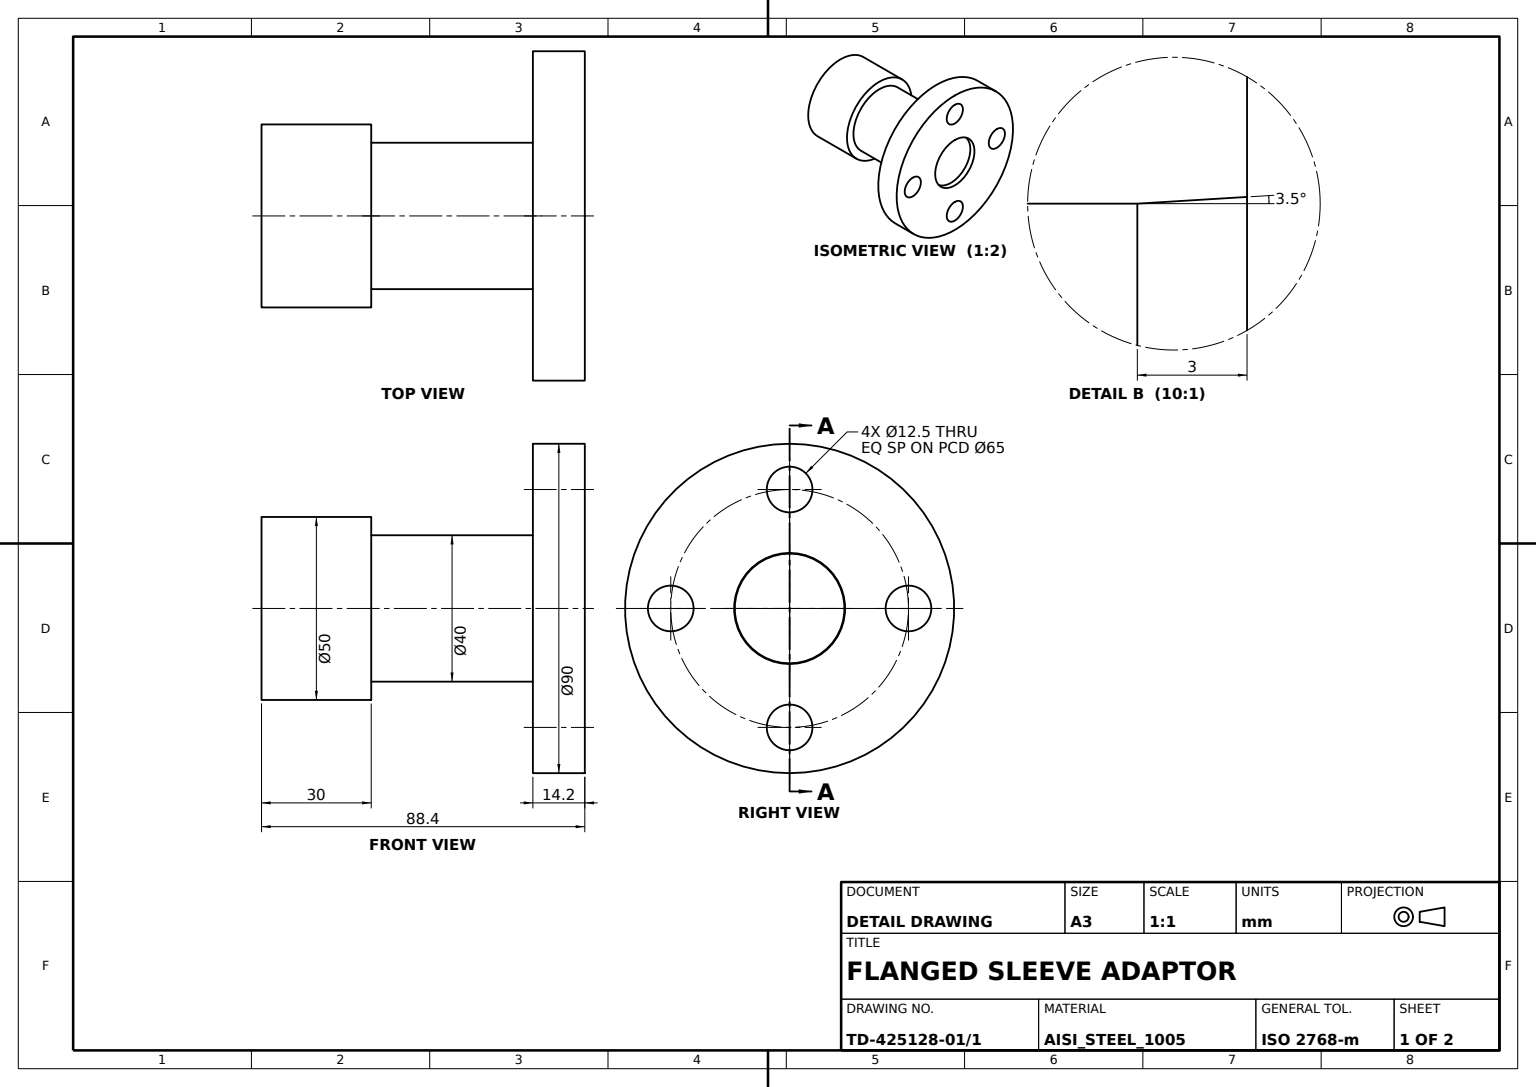
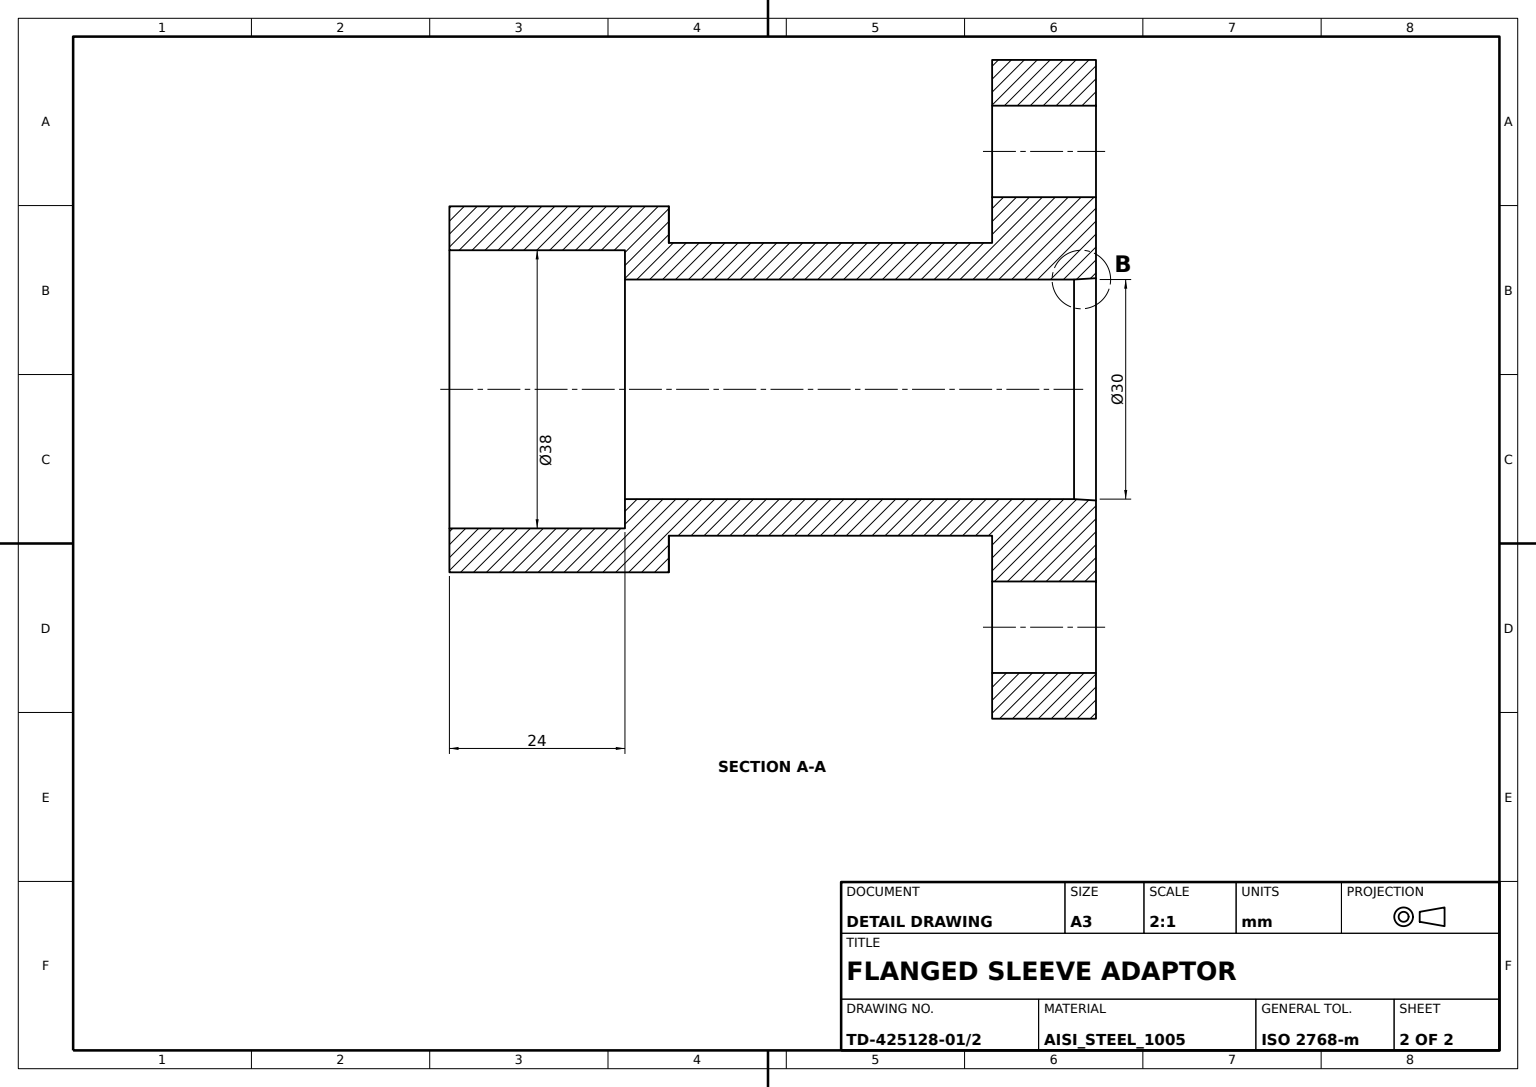
ISO-10303-21;
HEADER;
FILE_DESCRIPTION((''),'2;1');
FILE_NAME('','',(''),(''),'','','');
FILE_SCHEMA(('AUTOMOTIVE_DESIGN'));
ENDSEC;
DATA;
#1=APPLICATION_CONTEXT('');
#2=PRODUCT_CONTEXT('',#1,'mechanical');
#3=PRODUCT('','','',(#2));
#4=PRODUCT_DEFINITION_FORMATION('','',#3);
#5=PRODUCT_DEFINITION_CONTEXT('',#1,'design');
#6=PRODUCT_DEFINITION('','',#4,#5);
#7=PRODUCT_DEFINITION_SHAPE('','',#6);
#8=(LENGTH_UNIT()NAMED_UNIT(*)SI_UNIT(.MILLI.,.METRE.));
#9=(NAMED_UNIT(*)PLANE_ANGLE_UNIT()SI_UNIT($,.RADIAN.));
#10=(NAMED_UNIT(*)SI_UNIT($,.STERADIAN.)SOLID_ANGLE_UNIT());
#11=UNCERTAINTY_MEASURE_WITH_UNIT(LENGTH_MEASURE(0.005),#8,'distance_accuracy_value','');
#12=(GEOMETRIC_REPRESENTATION_CONTEXT(3)GLOBAL_UNCERTAINTY_ASSIGNED_CONTEXT((#11))GLOBAL_UNIT_ASSIGNED_CONTEXT((#8,#9,#10))REPRESENTATION_CONTEXT('',''));
#13=CARTESIAN_POINT('',(-58.4,0.,25.));
#14=VERTEX_POINT('',#13);
#15=CARTESIAN_POINT('',(-58.4,0.,0.));
#16=DIRECTION('',(-1.,0.,0.));
#17=DIRECTION('',(0.,0.,1.));
#18=AXIS2_PLACEMENT_3D('',#15,#16,#17);
#19=CIRCLE('',#18,25.);
#20=EDGE_CURVE('',#14,#14,#19,.T.);
#21=ORIENTED_EDGE('',*,*,#20,.F.);
#22=EDGE_LOOP('',(#21));
#23=FACE_BOUND('',#22,.T.);
#24=CARTESIAN_POINT('',(-58.4,0.,20.));
#25=VERTEX_POINT('',#24);
#26=CIRCLE('',#18,20.);
#27=EDGE_CURVE('',#25,#25,#26,.T.);
#28=ORIENTED_EDGE('',*,*,#27,.T.);
#29=EDGE_LOOP('',(#28));
#30=FACE_BOUND('',#29,.T.);
#31=AXIS2_PLACEMENT_3D('',#24,#16,#17);
#32=PLANE('',#31);
#33=ADVANCED_FACE('',(#23,#30),#32,.F.);
#34=CARTESIAN_POINT('',(-88.4,0.,25.));
#35=VERTEX_POINT('',#34);
#36=CARTESIAN_POINT('',(-88.4,0.,0.));
#37=AXIS2_PLACEMENT_3D('',#36,#16,#17);
#38=CIRCLE('',#37,25.);
#39=EDGE_CURVE('',#35,#35,#38,.T.);
#40=ORIENTED_EDGE('',*,*,#39,.F.);
#41=EDGE_LOOP('',(#40));
#42=FACE_BOUND('',#41,.T.);
#43=ORIENTED_EDGE('',*,*,#20,.T.);
#44=EDGE_LOOP('',(#43));
#45=FACE_BOUND('',#44,.T.);
#46=CARTESIAN_POINT('',(0.,0.,0.));
#47=AXIS2_PLACEMENT_3D('',#46,#16,#17);
#48=CYLINDRICAL_SURFACE('',#47,25.);
#49=ADVANCED_FACE('',(#42,#45),#48,.T.);
#50=CARTESIAN_POINT('',(0.,0.,45.));
#51=VERTEX_POINT('',#50);
#52=CIRCLE('',#47,45.);
#53=EDGE_CURVE('',#51,#51,#52,.T.);
#54=ORIENTED_EDGE('',*,*,#53,.T.);
#55=EDGE_LOOP('',(#54));
#56=FACE_BOUND('',#55,.T.);
#57=CARTESIAN_POINT('',(-14.2,0.,45.));
#58=VERTEX_POINT('',#57);
#59=CARTESIAN_POINT('',(-14.2,0.,0.));
#60=AXIS2_PLACEMENT_3D('',#59,#16,#17);
#61=CIRCLE('',#60,45.);
#62=EDGE_CURVE('',#58,#58,#61,.T.);
#63=ORIENTED_EDGE('',*,*,#62,.F.);
#64=EDGE_LOOP('',(#63));
#65=FACE_BOUND('',#64,.T.);
#66=CYLINDRICAL_SURFACE('',#47,45.);
#67=ADVANCED_FACE('',(#56,#65),#66,.T.);
#68=ORIENTED_EDGE('',*,*,#39,.T.);
#69=EDGE_LOOP('',(#68));
#70=FACE_BOUND('',#69,.T.);
#71=CARTESIAN_POINT('',(-88.4,19.,0.));
#72=VERTEX_POINT('',#71);
#73=DIRECTION('',(0.,1.,0.));
#74=AXIS2_PLACEMENT_3D('',#36,#16,#73);
#75=CIRCLE('',#74,19.);
#76=EDGE_CURVE('',#72,#72,#75,.T.);
#77=ORIENTED_EDGE('',*,*,#76,.F.);
#78=EDGE_LOOP('',(#77));
#79=FACE_BOUND('',#78,.T.);
#80=DIRECTION('',(1.,0.,0.));
#81=DIRECTION('',(0.,0.,-1.));
#82=AXIS2_PLACEMENT_3D('',#34,#80,#81);
#83=PLANE('',#82);
#84=ADVANCED_FACE('',(#70,#79),#83,.F.);
#85=CARTESIAN_POINT('',(-3.,0.,15.));
#86=VERTEX_POINT('',#85);
#87=CARTESIAN_POINT('',(-3.,0.,0.));
#88=AXIS2_PLACEMENT_3D('',#87,#16,#17);
#89=CIRCLE('',#88,15.);
#90=EDGE_CURVE('',#86,#86,#89,.F.);
#91=ORIENTED_EDGE('',*,*,#90,.T.);
#92=EDGE_LOOP('',(#91));
#93=FACE_BOUND('',#92,.T.);
#94=CARTESIAN_POINT('',(-64.4,0.,15.));
#95=VERTEX_POINT('',#94);
#96=CARTESIAN_POINT('',(-64.4,0.,0.));
#97=AXIS2_PLACEMENT_3D('',#96,#16,#17);
#98=CIRCLE('',#97,15.);
#99=EDGE_CURVE('',#95,#95,#98,.T.);
#100=ORIENTED_EDGE('',*,*,#99,.T.);
#101=EDGE_LOOP('',(#100));
#102=FACE_BOUND('',#101,.T.);
#103=CARTESIAN_POINT('',(24.,0.,0.));
#104=AXIS2_PLACEMENT_3D('',#103,#16,#17);
#105=CYLINDRICAL_SURFACE('',#104,15.);
#106=ADVANCED_FACE('',(#93,#102),#105,.F.);
#107=CARTESIAN_POINT('',(0.,0.,-26.25));
#108=VERTEX_POINT('',#107);
#109=CARTESIAN_POINT('',(0.,0.,-32.5));
#110=AXIS2_PLACEMENT_3D('',#109,#16,#17);
#111=CIRCLE('',#110,6.25);
#112=EDGE_CURVE('',#108,#108,#111,.T.);
#113=ORIENTED_EDGE('',*,*,#112,.F.);
#114=EDGE_LOOP('',(#113));
#115=FACE_BOUND('',#114,.T.);
#116=CARTESIAN_POINT('',(-14.2,0.,-38.75));
#117=VERTEX_POINT('',#116);
#118=CARTESIAN_POINT('',(-14.2,0.,-32.5));
#119=AXIS2_PLACEMENT_3D('',#118,#80,#81);
#120=CIRCLE('',#119,6.25);
#121=EDGE_CURVE('',#117,#117,#120,.F.);
#122=ORIENTED_EDGE('',*,*,#121,.T.);
#123=EDGE_LOOP('',(#122));
#124=FACE_BOUND('',#123,.T.);
#125=CARTESIAN_POINT('',(-38.2,0.,-32.5));
#126=AXIS2_PLACEMENT_3D('',#125,#80,#81);
#127=CYLINDRICAL_SURFACE('',#126,6.25);
#128=ADVANCED_FACE('',(#115,#124),#127,.F.);
#129=CARTESIAN_POINT('',(-64.4,19.,0.));
#130=VERTEX_POINT('',#129);
#131=AXIS2_PLACEMENT_3D('',#96,#16,#73);
#132=CIRCLE('',#131,19.);
#133=EDGE_CURVE('',#130,#130,#132,.F.);
#134=ORIENTED_EDGE('',*,*,#133,.F.);
#135=EDGE_LOOP('',(#134));
#136=FACE_BOUND('',#135,.T.);
#137=ORIENTED_EDGE('',*,*,#99,.F.);
#138=EDGE_LOOP('',(#137));
#139=FACE_BOUND('',#138,.T.);
#140=PLANE('',#97);
#141=ADVANCED_FACE('',(#136,#139),#140,.T.);
#142=ORIENTED_EDGE('',*,*,#27,.F.);
#143=EDGE_LOOP('',(#142));
#144=FACE_BOUND('',#143,.T.);
#145=CARTESIAN_POINT('',(-14.2,0.,20.));
#146=VERTEX_POINT('',#145);
#147=CIRCLE('',#60,20.);
#148=EDGE_CURVE('',#146,#146,#147,.T.);
#149=ORIENTED_EDGE('',*,*,#148,.T.);
#150=EDGE_LOOP('',(#149));
#151=FACE_BOUND('',#150,.T.);
#152=CYLINDRICAL_SURFACE('',#47,20.);
#153=ADVANCED_FACE('',(#144,#151),#152,.T.);
#154=CARTESIAN_POINT('',(0.,0.,38.75));
#155=VERTEX_POINT('',#154);
#156=CARTESIAN_POINT('',(0.,0.,32.5));
#157=AXIS2_PLACEMENT_3D('',#156,#16,#17);
#158=CIRCLE('',#157,6.25);
#159=EDGE_CURVE('',#155,#155,#158,.T.);
#160=ORIENTED_EDGE('',*,*,#159,.T.);
#161=EDGE_LOOP('',(#160));
#162=FACE_BOUND('',#161,.T.);
#163=CARTESIAN_POINT('',(0.,32.5,6.25));
#164=VERTEX_POINT('',#163);
#165=CARTESIAN_POINT('',(0.,32.5,0.));
#166=AXIS2_PLACEMENT_3D('',#165,#16,#17);
#167=CIRCLE('',#166,6.25);
#168=EDGE_CURVE('',#164,#164,#167,.T.);
#169=ORIENTED_EDGE('',*,*,#168,.T.);
#170=EDGE_LOOP('',(#169));
#171=FACE_BOUND('',#170,.T.);
#172=ORIENTED_EDGE('',*,*,#53,.F.);
#173=EDGE_LOOP('',(#172));
#174=FACE_BOUND('',#173,.T.);
#175=CARTESIAN_POINT('',(0.,-32.5,6.25));
#176=VERTEX_POINT('',#175);
#177=CARTESIAN_POINT('',(0.,-32.5,0.));
#178=AXIS2_PLACEMENT_3D('',#177,#16,#17);
#179=CIRCLE('',#178,6.25);
#180=EDGE_CURVE('',#176,#176,#179,.T.);
#181=ORIENTED_EDGE('',*,*,#180,.T.);
#182=EDGE_LOOP('',(#181));
#183=FACE_BOUND('',#182,.T.);
#184=CARTESIAN_POINT('',(0.,0.,15.183488));
#185=VERTEX_POINT('',#184);
#186=CIRCLE('',#47,15.183488);
#187=EDGE_CURVE('',#185,#185,#186,.T.);
#188=ORIENTED_EDGE('',*,*,#187,.T.);
#189=EDGE_LOOP('',(#188));
#190=FACE_BOUND('',#189,.T.);
#191=ORIENTED_EDGE('',*,*,#112,.T.);
#192=EDGE_LOOP('',(#191));
#193=FACE_BOUND('',#192,.T.);
#194=PLANE('',#47);
#195=ADVANCED_FACE('',(#162,#171,#174,#183,#190,#193),#194,.F.);
#196=ORIENTED_EDGE('',*,*,#180,.F.);
#197=EDGE_LOOP('',(#196));
#198=FACE_BOUND('',#197,.T.);
#199=CARTESIAN_POINT('',(-14.2,-32.5,-6.25));
#200=VERTEX_POINT('',#199);
#201=CARTESIAN_POINT('',(-14.2,-32.5,0.));
#202=AXIS2_PLACEMENT_3D('',#201,#80,#81);
#203=CIRCLE('',#202,6.25);
#204=EDGE_CURVE('',#200,#200,#203,.F.);
#205=ORIENTED_EDGE('',*,*,#204,.T.);
#206=EDGE_LOOP('',(#205));
#207=FACE_BOUND('',#206,.T.);
#208=CARTESIAN_POINT('',(-38.2,-32.5,0.));
#209=AXIS2_PLACEMENT_3D('',#208,#80,#81);
#210=CYLINDRICAL_SURFACE('',#209,6.25);
#211=ADVANCED_FACE('',(#198,#207),#210,.F.);
#212=ORIENTED_EDGE('',*,*,#168,.F.);
#213=EDGE_LOOP('',(#212));
#214=FACE_BOUND('',#213,.T.);
#215=CARTESIAN_POINT('',(-14.2,32.5,-6.25));
#216=VERTEX_POINT('',#215);
#217=CARTESIAN_POINT('',(-14.2,32.5,0.));
#218=AXIS2_PLACEMENT_3D('',#217,#80,#81);
#219=CIRCLE('',#218,6.25);
#220=EDGE_CURVE('',#216,#216,#219,.F.);
#221=ORIENTED_EDGE('',*,*,#220,.T.);
#222=EDGE_LOOP('',(#221));
#223=FACE_BOUND('',#222,.T.);
#224=CARTESIAN_POINT('',(-38.2,32.5,0.));
#225=AXIS2_PLACEMENT_3D('',#224,#80,#81);
#226=CYLINDRICAL_SURFACE('',#225,6.25);
#227=ADVANCED_FACE('',(#214,#223),#226,.F.);
#228=ORIENTED_EDGE('',*,*,#133,.T.);
#229=EDGE_LOOP('',(#228));
#230=FACE_BOUND('',#229,.T.);
#231=ORIENTED_EDGE('',*,*,#76,.T.);
#232=EDGE_LOOP('',(#231));
#233=FACE_BOUND('',#232,.T.);
#234=CYLINDRICAL_SURFACE('',#97,19.);
#235=ADVANCED_FACE('',(#230,#233),#234,.F.);
#236=ORIENTED_EDGE('',*,*,#148,.F.);
#237=EDGE_LOOP('',(#236));
#238=FACE_BOUND('',#237,.T.);
#239=ORIENTED_EDGE('',*,*,#121,.F.);
#240=EDGE_LOOP('',(#239));
#241=FACE_BOUND('',#240,.T.);
#242=CARTESIAN_POINT('',(-14.2,0.,26.25));
#243=VERTEX_POINT('',#242);
#244=CARTESIAN_POINT('',(-14.2,0.,32.5));
#245=AXIS2_PLACEMENT_3D('',#244,#80,#81);
#246=CIRCLE('',#245,6.25);
#247=EDGE_CURVE('',#243,#243,#246,.F.);
#248=ORIENTED_EDGE('',*,*,#247,.F.);
#249=EDGE_LOOP('',(#248));
#250=FACE_BOUND('',#249,.T.);
#251=ORIENTED_EDGE('',*,*,#204,.F.);
#252=EDGE_LOOP('',(#251));
#253=FACE_BOUND('',#252,.T.);
#254=ORIENTED_EDGE('',*,*,#62,.T.);
#255=EDGE_LOOP('',(#254));
#256=FACE_BOUND('',#255,.T.);
#257=ORIENTED_EDGE('',*,*,#220,.F.);
#258=EDGE_LOOP('',(#257));
#259=FACE_BOUND('',#258,.T.);
#260=AXIS2_PLACEMENT_3D('',#57,#80,#81);
#261=PLANE('',#260);
#262=ADVANCED_FACE('',(#238,#241,#250,#253,#256,#259),#261,.F.);
#263=ORIENTED_EDGE('',*,*,#187,.F.);
#264=EDGE_LOOP('',(#263));
#265=FACE_BOUND('',#264,.T.);
#266=ORIENTED_EDGE('',*,*,#90,.F.);
#267=EDGE_LOOP('',(#266));
#268=FACE_BOUND('',#267,.T.);
#269=AXIS2_PLACEMENT_3D('',#87,#80,#81);
#270=CONICAL_SURFACE('',#269,15.,0.061086524);
#271=ADVANCED_FACE('',(#265,#268),#270,.F.);
#272=ORIENTED_EDGE('',*,*,#247,.T.);
#273=EDGE_LOOP('',(#272));
#274=FACE_BOUND('',#273,.T.);
#275=ORIENTED_EDGE('',*,*,#159,.F.);
#276=EDGE_LOOP('',(#275));
#277=FACE_BOUND('',#276,.T.);
#278=CARTESIAN_POINT('',(-38.2,0.,32.5));
#279=AXIS2_PLACEMENT_3D('',#278,#80,#81);
#280=CYLINDRICAL_SURFACE('',#279,6.25);
#281=ADVANCED_FACE('',(#274,#277),#280,.F.);
#282=CLOSED_SHELL('',(#33,#49,#67,#84,#106,#128,#141,#153,#195,#211,#227,#235,#262,#271,#281));
#283=MANIFOLD_SOLID_BREP('',#282);
#284=ADVANCED_BREP_SHAPE_REPRESENTATION('',(#283),#12);
#285=SHAPE_DEFINITION_REPRESENTATION(#7,#284);
ENDSEC;
END-ISO-10303-21;
